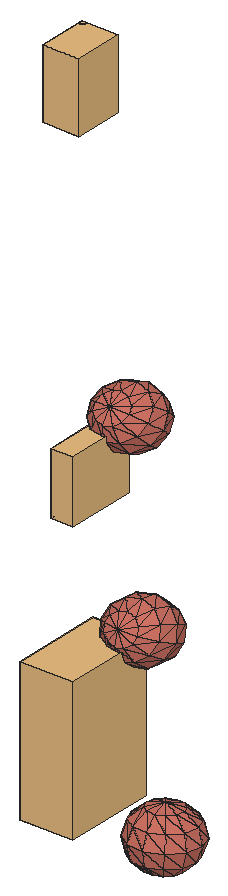
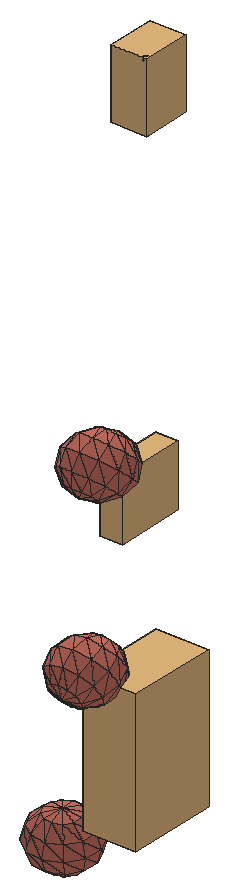
# SketchUp Ruby script. Lengths in inches.
U = 1.inch
M = Sketchup.active_model
def pt(a) = Geom::Point3d.new(a.map { |v| v * U })
def face(e, loops, mat)
  f = e.add_face(loops[0].map { |a| pt(a) })
  loops[1..].each { |l| e.add_face(l.map { |a| pt(a) }).erase! }
  f.material = f.back_material = mat if mat
  f
end
# faces: each face lists its corners as indices into pts; further lists are holes
def faces(e, pts, list, mat = nil) = list.each { |f| face(e, (f[0].is_a?(Array) ? f : [f]).map { |l| l.map { |i| pts[i] } }, mat) }
# xy, xz, yz: faces in a plane at the given z, y or x. An outline is a flat list of corners, or four numbers for a rectangle; further outlines are holes
def ring(l) = l.size == 4 ? [[l[0], l[1]], [l[2], l[1]], [l[2], l[3]], [l[0], l[3]]] : l.each_slice(2).to_a
def flat(e, list, mat, &to3) = list.each { |f| face(e, (f[0].is_a?(Array) ? f : [f]).map { |l| ring(l).map { |u, v| to3.(u, v) } }, mat) }
def xy(e, z, list, mat = nil) = flat(e, list, mat) { |x, y| [x, y, z] }
def xz(e, y, list, mat = nil) = flat(e, list, mat) { |x, z| [x, y, z] }
def yz(e, x, list, mat = nil) = flat(e, list, mat) { |y, z| [x, y, z] }
def lines(e, pts, list) = list.each { |a, b| e.add_line(pt(pts[a]), pt(pts[b])) }
# prism: a flat outline (further loops are holes) pulled along v
def prism(e, loops, v, mat = nil)
  f = face(e, loops, mat); d = Geom::Vector3d.new(v.map { |x| x * U })
  f.pushpull(f.normal.samedirection?(d) ? d.length : -d.length)
end
def box(e, o, s, mat = nil) = prism(e, [[o, [o[0] + s[0], o[1], o[2]], [o[0] + s[0], o[1] + s[1], o[2]], [o[0], o[1] + s[1], o[2]]]], [0, 0, s[2]], mat)
def at(x, y, z, deg = 0) = Geom::Transformation.translation(pt([x, y, z])) * Geom::Transformation.rotation(ORIGIN, Z_AXIS, deg.degrees)
def axes(o, x, y, z) = Geom::Transformation.new([*x, 0, *y, 0, *z, 0, *pt(o).to_a, 1])
def part(name) = M.definitions.add(name)
# library, detail: a bought-in or finely detailed component or shape, given as its bounding box
def library(name, o, s) = part(name).tap { |d| box(d.entities, o, s) }
def detail(e, o, s) = box(e.add_group.entities, o, s)
def put(e, d, t, mat = nil) = e.add_instance(d, t).tap { |i| i.material = mat if mat }
def group(e, t, mat = nil) = e.add_group.tap { |g| g.transformation = t; g.material = mat if mat }.entities
root = M.entities
M.materials.add("green").color = [174, 139, 102]
M.materials.add("vio").color = [206, 114, 100]
c1 = library("3DGeom~25_Defintion",[-351.97,-500,-258.4],[703.94,1000,516.8])
c2 = part("3DGeom~26_Defintion")
p = [[-344.73,487.39,-243.89],[-293.86,494.46,-251.4],[-311.18,491.2,-258.4],[-344.73,487.39,-243.89],[-311.18,491.2,-258.4],[-329.79,488.61,-255.65],
  [-344.73,487.39,-243.89],[-282.49,497.51,-236.53],[-293.86,494.46,-251.4],[-344.73,487.39,-243.89],[-351.97,487.85,-226.26],[-349.59,489.88,-207.5],
  [-344.73,487.39,-243.89],[-349.59,489.88,-207.5],[-338.22,492.93,-192.625],[-344.73,487.39,-243.89],[-280.11,499.54,-217.76],[-282.49,497.51,-236.53],
  [-344.73,487.39,-243.89],[-302.29,498.77,-188.375],[-287.36,500,-200.14],[-344.73,487.39,-243.89],[-287.36,500,-200.14],[-280.11,499.54,-217.76],
  [-344.73,487.39,-243.89],[-338.22,492.93,-192.625],[-320.91,496.1875,-185.625],[-344.73,487.39,-243.89],[-320.91,496.1875,-185.625],[-302.29,498.77,-188.375],
  [300.11,-500,207.2],[314.12,-496.86,194.8],[330.21,-489.05,190.33],[351.97,-468.47,207.5],[300.11,-500,207.2],[330.21,-489.05,190.33],
  [351.97,-468.47,207.5],[330.21,-489.05,190.33],[344.06,-478.66,194.98],[291.79,-490.37,241.23],[300.11,-500,207.2],[313.56,-469.79,258.4],
  [300.11,-500,207.2],[291.79,-490.37,241.23],[291.94,-497.625,224.19],[343.65,-458.84,241.54],[300.11,-500,207.2],[351.97,-468.47,207.5],
  [313.56,-469.79,258.4],[300.11,-500,207.2],[343.65,-458.84,241.54],[343.65,-458.84,241.54],[351.97,-468.47,207.5],[351.82,-461.21,224.54],
  [291.79,-490.37,241.23],[313.56,-469.79,258.4],[299.7,-480.18,253.76],[313.56,-469.79,258.4],[343.65,-458.84,241.54],[329.64,-461.98,253.93]]
faces(c2.entities,p,[[0,1,2],[3,4,5],[6,7,8],[9,10,11],[12,13,14],[15,16,17],[18,19,20],[21,22,23],
  [24,25,26],[27,28,29],[30,31,32],[33,34,35],[36,37,38],[39,40,41],[42,43,44],[45,46,47],
  [48,49,50],[51,52,53],[54,55,56],[57,58,59]],"green")
c3 = library("3DGeom~17_Defintion",[-322.12,-500,-186.09],[644.24,1000,372.18])
c4 = part("3DGeom~18_Defintion")
p = [[292.74,-500,-165.38],[307.55,-495.14,-174.52],[291.14,-497.07,-147.46],[307.55,-495.14,-174.52],[292.74,-500,-165.38],[299.25,-498.4,-172.01],
  [291.14,-497.07,-147.46],[307.55,-495.14,-174.52],[304.35,-489.29,-138.68],[304.35,-489.29,-138.68],[307.55,-495.14,-174.52],[319.15,-484.43,-147.83],
  [307.55,-495.14,-174.52],[315.42,-491.1,-172.22],[320.75,-487.36,-165.74],[320.75,-487.36,-165.74],[319.15,-484.43,-147.83],[320.75,-487.36,-165.74],
  [322.12,-484.92,-156.8125],[292.74,-500,-165.38],[291.14,-497.07,-147.46],[289.78,-499.51,-156.39],[304.35,-489.29,-138.68],[319.15,-484.43,-147.83],
  [312.65,-486.03,-141.19],[291.14,-497.07,-147.46],[304.35,-489.29,-138.68],[296.48,-493.33,-140.98],[-309.07,495.99,151.67],[-322.12,484.07,169.09],
  [-318.39,482.74,177.66],[-309.07,495.99,151.67],[-318.39,482.74,177.66],[-311.33,483.72,183.88],[-309.07,495.99,151.67],[-311.33,483.72,183.88],
  [-302.83,486.75,186.09],[-309.07,495.99,151.67],[-321.51,487.36,160.45],[-322.12,484.07,169.09],[-309.07,495.99,151.67],[-302.83,486.75,186.09],
  [-295.16,491.02,183.67],[-309.07,495.99,151.67],[-316.73,491.72,154.08],[-321.51,487.36,160.45],[-309.07,495.99,151.67],[-295.16,491.02,183.67],
  [-290.38,495.38,177.3],[-309.07,495.99,151.67],[-290.38,495.38,177.3],[-289.78,498.67,168.67],[-309.07,495.99,151.67],[-289.78,498.67,168.67],
  [-293.5,500,160.09],[-309.07,495.99,151.67],[-293.5,500,160.09],[-300.5625,499.02,153.87]]
faces(c4.entities,p,[[0,1,2],[3,4,5],[6,7,8],[9,10,11],[12,13,14],[11,10,15],[16,17,18],[19,20,21],
  [22,23,24],[25,26,27],[28,29,30],[31,32,33],[34,35,36],[37,38,39],[40,41,42],[43,44,45],
  [46,47,48],[49,50,51],[52,53,54],[55,56,57]],"green")
c5 = library("3DGeom~21_Defintion",[-500,-446.39,-160.99],[1000,892.78,321.97])
c6 = part("3DGeom~22_Defintion")
p = [[448.91,-442.9,-142.17],[471.3125,-423.55,-160.99],[450.7,-444.07,-105.16],[450.7,-444.07,-105.16],[471.3125,-423.55,-160.99],[474.89,-425.89,-86.96],
  [471.3125,-423.55,-160.99],[448.91,-442.9,-142.17],[458.1,-434.54,-155.85],[474.89,-425.89,-86.96],[471.3125,-423.55,-160.99],[497.29,-406.54,-105.77],
  [471.3125,-423.55,-160.99],[485,-412.87,-156.2],[495.5,-405.37,-142.78],[471.3125,-423.55,-160.99],[495.5,-405.37,-142.78],[495.5,-405.37,-142.78],
  [500,-403.05,-124.32],[448.91,-442.9,-142.17],[450.7,-444.07,-105.16],[446.2,-446.39,-123.62],[474.89,-425.89,-86.96],[488.1,-414.9,-92.09],
  [450.7,-444.07,-105.16],[474.89,-425.89,-86.96],[461.21,-436.57,-91.74],[-483.76,433.75,98.79],[-496.54,399.82,130.23],[-485.88,396.59,145.74],
  [-483.76,433.75,98.79],[-485.88,396.59,145.74],[-470.87,400.03,156.99],[-483.76,433.75,98.79],[-500,408.86,114.64],[-496.54,399.82,130.23],
  [-483.76,433.75,98.79],[-470.87,400.03,156.99],[-455.53,409.22,160.98],[-483.76,433.75,98.79],[-495.32,421.28,103.125],[-483.76,433.75,98.79],
  [-455.53,409.22,160.98],[-443.97,421.7,156.64],[-483.76,433.75,98.79],[-443.97,421.7,156.64],[-439.29,434.12,145.13],[-483.76,433.75,98.79],
  [-442.75,443.16,129.53],[-453.41,446.39,114.03],[-483.76,433.75,98.79],[-453.41,446.39,114.03],[-468.42,442.95,102.78],[-483.76,433.75,98.79],
  [-439.29,434.12,145.13],[-442.75,443.16,129.53]]
faces(c6.entities,p,[[0,1,2],[3,4,5],[6,7,8],[9,10,11],[12,13,14],[11,15,16],[11,17,18],[19,20,21],
  [22,11,23],[24,25,26],[27,28,29],[30,31,32],[33,34,35],[36,37,38],[39,40,34],[41,42,43],
  [44,45,46],[47,48,49],[50,51,52],[53,54,55]],"green")
c7 = part("3DGeom~225_Defintion")
p = [[77.58,-12.43,-500],[-128.33,-244.69,-395.82],[-181.28,-36.33,-470.68],[95.84,-224,-421.21],[315.65,14.8,-395.34],[38.53,202.47,-444.81],
  [244.7,226.05,-354.18],[-310.44,-256.96,-261.21],[-391.56,-50.49,-315.24],[-310.44,-256.96,-261.21],[-185.65,181.77,-419.42],[-391.56,-50.49,-315.24],
  [-10.85,363.12,-270.44],[108.1875,376.73,-218.11],[-10.85,363.12,-270.44],[108.1875,376.73,-218.11],[-41,-387.49,-214.9],[88.43,-375.54,-229.56],
  [-41,-387.49,-214.9],[302.01,-200.41,-330.58],[-391.56,-50.49,-315.24],[-367.76,169.5,-284.8125],[-140.27,351.16,-255.78],[-367.76,169.5,-284.8125],
  [-10.85,363.12,-270.44],[-140.27,351.16,-255.78],[-128.33,-244.69,-395.82],[-146.14,-394.58,-137.18],[-310.44,-256.96,-261.21],[-128.33,-244.69,-395.82],
  [-41,-387.49,-214.9],[469.13,38.07,-184.76],[302.01,-200.41,-330.58],[315.65,14.8,-395.34],[377.625,246.2,-171.81],[315.65,14.8,-395.34],
  [244.7,226.05,-354.18],[377.625,246.2,-171.81],[315.65,14.8,-395.34],[184.93,388.36,-112.82],[244.7,226.05,-354.18],[108.1875,376.73,-218.11],
  [377.625,246.2,-171.81],[244.7,226.05,-354.18],[207.46,-361.93,-177.23],[434.94,-180.27,-148.2],[207.46,-361.93,-177.23],[302.01,-200.41,-330.58],
  [302.01,-200.41,-330.58],[-391.56,-50.49,-315.24],[-401.6875,-257.51,-53.44],[-496.92,-51.13,-75.34],[-310.44,-256.96,-261.21],[-367.76,169.5,-284.8125],
  [-459,168.95,-77.05],[-245.41,344.08,-178.0625],[-140.27,351.16,-255.78],[-367.76,169.5,-284.8125],[-245.41,344.08,-178.0625],[-10.85,363.12,-270.44],
  [-140.27,351.16,-255.78],[-57.32,426.47,-23.6],[-310.44,-256.96,-261.21],[-198.82,-394.9,-17.23],[-401.6875,-257.51,-53.44],[-310.44,-256.96,-261.21],
  [-245.41,344.08,-178.0625],[88.43,-375.54,-229.56],[57.32,-426.47,23.6],[88.43,-375.54,-229.56],[207.46,-361.93,-177.23],[496.92,51.13,75.34],
  [401.6875,257.51,53.44],[377.625,246.2,-171.81],[401.6875,257.51,53.44],[-245.41,344.08,-178.0625],[-298.1,343.77,-58.11],[-298.1,343.77,-58.11],
  [207.46,-361.93,-177.23],[284.2,-350.3,-71.9375],[284.2,-350.3,-71.9375],[207.46,-361.93,-177.23],[198.82,394.9,17.23],[401.6875,257.51,53.44],
  [459,-168.95,77.05],[-469.13,-38.07,184.76],[-434.94,180.27,148.2],[-298.1,343.77,-58.11],[-377.625,-246.2,171.81],[284.2,-350.3,-71.9375],
  [298.1,-343.77,58.11],[298.1,-343.77,58.11],[-298.1,343.77,-58.11],[-284.2,350.3,71.9375],[-284.2,350.3,71.9375],[-401.6875,-257.51,-53.44],
  [-184.93,-388.36,112.82],[-401.6875,-257.51,-53.44],[-377.625,-246.2,171.81],[-207.46,361.93,177.23],[-88.43,375.54,229.56],[41,387.49,214.9],
  [146.14,394.58,137.18],[-108.1875,-376.73,218.11],[10.85,-363.12,270.44],[-108.1875,-376.73,218.11],[140.27,-351.16,255.78],[10.85,-363.12,270.44],
  [298.1,-343.77,58.11],[245.41,-344.08,178.0625],[245.41,-344.08,178.0625],[140.27,-351.16,255.78],[310.44,256.96,261.21],[401.6875,257.51,53.44],
  [310.44,256.96,261.21],[367.76,-169.5,284.8125],[245.41,-344.08,178.0625],[-284.2,350.3,71.9375],[-302.01,200.41,330.58],[-284.2,350.3,71.9375],
  [-302.01,200.41,330.58],[-207.46,361.93,177.23],[391.56,50.49,315.24],[310.44,256.96,261.21],[-377.625,-246.2,171.81],[-108.1875,-376.73,218.11],
  [-315.65,-14.8,395.34],[-315.65,-14.8,395.34],[-302.01,200.41,330.58],[-377.625,-246.2,171.81],[-108.1875,-376.73,218.11],[-244.7,-226.05,354.18],
  [-244.7,-226.05,354.18],[-207.46,361.93,177.23],[-302.01,200.41,330.58],[-95.84,224,421.21],[-207.46,361.93,177.23],[-88.43,375.54,229.56],
  [185.65,-181.77,419.42],[140.27,-351.16,255.78],[245.41,-344.08,178.0625],[245.41,-344.08,178.0625],[367.76,-169.5,284.8125],[-244.7,-226.05,354.18],
  [-315.65,-14.8,395.34],[-88.43,375.54,229.56],[128.33,244.69,395.82],[41,387.49,214.9],[128.33,244.69,395.82],[-244.7,-226.05,354.18],
  [-108.1875,-376.73,218.11],[10.85,-363.12,270.44],[-88.43,375.54,229.56],[128.33,244.69,395.82],[-38.53,-202.47,444.81],[128.33,244.69,395.82],
  [391.56,50.49,315.24],[310.44,256.96,261.21],[181.28,36.33,470.68],[367.76,-169.5,284.8125],[367.76,-169.5,284.8125],[391.56,50.49,315.24],
  [128.33,244.69,395.82],[391.56,50.49,315.24],[-315.65,-14.8,395.34],[-77.58,12.43,500],[128.33,244.69,395.82]]
faces(c7.entities,p,[[0,1,2],[0,3,1],[4,3,0],[5,0,2],[6,0,5],[6,4,0],[2,7,8],[2,1,9],
  [10,2,11],[5,2,10],[12,5,10],[13,5,14],[15,6,5],[3,16,1],[3,17,18],[19,17,3],
  [4,19,3],[10,20,21],[22,10,23],[24,10,25],[26,27,28],[29,30,27],[31,32,33],[34,35,36],
  [37,31,38],[39,40,41],[39,42,43],[19,44,17],[45,46,47],[31,45,48],[49,50,51],[49,52,50],
  [53,49,51],[53,51,54],[55,53,54],[56,57,58],[59,60,61],[41,59,61],[62,63,64],[65,27,63],
  [60,66,61],[30,67,68],[69,70,68],[39,41,61],[27,30,68],[71,45,31],[72,31,73],[74,71,31],
  [75,54,76],[66,77,61],[78,79,68],[45,80,81],[82,42,39],[82,83,42],[84,80,45],[71,84,45],
  [63,27,68],[82,39,61],[54,51,85],[54,85,86],[87,54,86],[51,50,88],[51,88,85],[89,90,68],
  [84,91,80],[92,86,93],[77,94,61],[95,63,96],[97,96,98],[94,99,61],[99,100,61],[100,101,61],
  [101,102,61],[102,82,61],[96,63,68],[102,83,82],[103,96,68],[104,105,68],[106,107,68],[108,109,68],
  [110,111,68],[112,71,113],[102,114,83],[115,116,91],[115,91,84],[117,86,118],[119,120,121],[122,84,71],
  [123,122,71],[122,115,84],[124,96,125],[101,114,102],[86,85,126],[86,127,128],[129,130,131],[85,88,132],
  [133,134,135],[136,135,137],[138,139,140],[138,141,142],[85,143,144],[145,146,147],[101,148,114],[149,150,151],
  [152,135,153],[154,151,139],[154,139,138],[155,156,157],[149,151,154],[158,138,159],[158,160,161],[162,158,163],
  [134,164,165],[134,165,135],[164,149,154],[164,154,165],[135,158,166],[165,154,138],[165,138,158],[135,165,158]],"vio")
c8 = part("3DGeom~195_Defintion")
p = [[166.45,-153.95,-435.25],[-186.98,-146.09,-430.65],[-6.51,0,-500],[325.5,12.77,-379.3],[-335.26,-12.77,-370.7],[-177.72,153.95,-430.77],
  [175.71,146.09,-435.37],[397.32,176.07,-221.71],[27.43,279.42,-375.42],[310.84,253.04,-254.09],[27.43,279.42,-375.42],[397.32,176.07,-221.71],
  [310.84,253.04,-254.09],[-37.19,-279.42,-374.58],[294.8125,-266.65,-253.88],[436.66,-84.83,-222.23],[436.66,-84.83,-222.23],[-442.29,84.83,-210.79],
  [-442.29,84.83,-210.79],[-301.32,266.65,-246.12],[27.43,279.42,-375.42],[-301.32,266.65,-246.12],[-317.35,-253.04,-245.91],[-402.96,-176.07,-211.3],
  [-402.96,-176.07,-211.3],[461.5,119.72,-131.03],[436.66,-84.83,-222.23],[325.5,12.77,-379.3],[325.5,12.77,-379.3],[397.32,176.07,-221.71],
  [310.84,253.04,-254.09],[27.43,279.42,-375.42],[225.23,330.02,-219.47],[27.43,279.42,-375.42],[-301.32,266.65,-246.12],[-79.61,377.03,-215.51],
  [225.23,330.02,-219.47],[27.43,279.42,-375.42],[-79.61,377.03,-215.51],[73.97,-377.02,-217.51],[-230.87,-330.02,-213.54],[-37.19,-279.42,-374.58],
  [73.97,-377.02,-217.51],[-230.87,-330.02,-213.54],[-335.26,-12.77,-370.7],[-402.96,-176.07,-211.3],[-464.76,-119.72,-118.97],[-335.26,-12.77,-370.7],
  [-442.29,84.83,-210.79],[310.84,253.04,-254.09],[362.6875,292.19,-4.72],[225.23,330.02,-219.47],[344.18,-307.91,-4.48],[73.97,-377.02,-217.51],
  [294.8125,-266.65,-253.88],[479.41,-120.56,-6.24],[344.18,-307.91,-4.48],[294.8125,-266.65,-253.88],[294.8125,-266.65,-253.88],[-301.32,266.65,-246.12],
  [-479.41,120.56,6.24],[-301.32,266.65,-246.12],[-344.18,307.91,4.48],[-301.32,266.65,-246.12],[-344.18,307.91,4.48],[-317.35,-253.04,-245.91],
  [-230.87,-330.02,-213.54],[-362.6875,-292.19,4.72],[-317.35,-253.04,-245.91],[-362.6875,-292.19,4.72],[486.1875,99.09,-6.33],[163.4375,386.37,-127.15],
  [362.6875,292.19,-4.72],[116.72,-412.75,-1.52],[-166.69,-386.37,-122.85],[73.97,-377.02,-217.51],[344.18,-307.91,-4.48],[73.97,-377.02,-217.51],
  [73.97,-377.02,-217.51],[-230.87,-330.02,-213.54],[-116.72,412.75,1.52],[-230.87,-330.02,-213.54],[-362.6875,-292.19,4.72],[-362.6875,-292.19,4.72],
  [-486.1875,-99.09,6.33],[142.01,407,-1.85],[362.6875,292.19,-4.72],[-142.01,-407,1.85],[-362.6875,-292.19,4.72],[464.76,119.72,118.97],
  [442.29,-84.83,210.79],[402.96,176.07,211.3],[317.35,253.04,245.91],[230.87,330.02,213.54],[166.69,386.37,122.85],[362.6875,292.19,-4.72],
  [230.87,330.02,213.54],[362.6875,292.19,-4.72],[301.32,-266.65,246.12],[344.18,-307.91,-4.48],[301.32,-266.65,246.12],[-73.97,377.02,217.51],
  [79.61,-377.03,215.51],[301.32,-266.65,246.12],[-294.8125,266.65,253.88],[-294.8125,266.65,253.88],[-163.4375,-386.37,127.15],[-344.18,307.91,4.48],
  [-436.66,84.83,222.23],[-344.18,307.91,4.48],[-436.66,84.83,222.23],[-294.8125,266.65,253.88],[-225.24,-330.02,219.47],[-225.24,-330.02,219.47],
  [-310.84,-253.04,254.09],[-362.6875,-292.19,4.72],[-461.5,-119.72,131.03],[-362.6875,-292.19,4.72],[-397.32,-176.07,221.71],[-362.6875,-292.19,4.72],
  [-310.84,-253.04,254.09],[-397.32,-176.07,221.71],[-362.6875,-292.19,4.72],[-436.66,84.83,222.23],[37.19,279.42,374.58],[37.19,279.42,374.58],
  [230.87,330.02,213.54],[-27.43,-279.42,375.42],[-27.43,-279.42,375.42],[-436.66,84.83,222.23],[-397.32,-176.07,221.71],[335.26,12.77,370.7],
  [301.32,-266.65,246.12],[442.29,-84.83,210.79],[335.26,12.77,370.7],[317.35,253.04,245.91],[335.26,12.77,370.7],[402.96,176.07,211.3],
  [230.87,330.02,213.54],[37.19,279.42,374.58],[186.98,146.09,430.65],[230.87,330.02,213.54],[317.35,253.04,245.91],[177.72,-153.95,430.77],
  [-27.43,-279.42,375.42],[79.61,-377.03,215.51],[79.61,-377.03,215.51],[301.32,-266.65,246.12],[-73.97,377.02,217.51],[-294.8125,266.65,253.88],
  [-166.45,153.95,435.25],[-73.97,377.02,217.51],[-175.71,-146.09,435.37],[-310.84,-253.04,254.09],[-225.24,-330.02,219.47],[-225.24,-330.02,219.47],
  [-325.5,-12.77,379.3],[-397.32,-176.07,221.71],[-436.66,84.83,222.23],[-397.32,-176.07,221.71],[-325.5,-12.77,379.3],[-436.66,84.83,222.23],
  [317.35,253.04,245.91],[335.26,12.77,370.7],[335.26,12.77,370.7],[301.32,-266.65,246.12],[335.26,12.77,370.7],[6.51,0,500]]
faces(c8.entities,p,[[0,1,2],[3,0,2],[2,1,4],[2,4,5],[6,2,5],[3,2,6],[7,3,6],[6,5,8],
  [9,6,10],[11,6,12],[0,13,1],[14,13,0],[15,14,0],[16,0,3],[5,4,17],[5,18,19],
  [20,5,21],[13,22,1],[1,22,23],[1,24,4],[25,26,27],[25,28,29],[30,31,32],[33,34,35],
  [36,37,38],[39,40,41],[14,42,13],[13,43,22],[44,45,46],[47,46,48],[29,49,50],[49,51,50],
  [52,53,54],[55,56,57],[55,58,26],[59,48,60],[61,60,62],[38,63,64],[65,66,67],[45,68,69],
  [70,55,26],[70,26,25],[25,29,50],[36,71,72],[36,38,71],[73,74,75],[76,73,77],[78,74,79],
  [38,64,80],[71,38,80],[81,74,82],[46,45,83],[48,46,84],[48,84,60],[70,25,50],[71,85,86],
  [71,80,85],[73,87,74],[74,87,82],[84,46,88],[89,55,70],[89,70,50],[90,56,55],[89,90,55],
  [91,89,50],[92,91,50],[93,92,50],[85,94,95],[94,96,97],[98,73,99],[90,100,56],[85,80,101],
  [85,101,94],[102,87,73],[103,102,73],[80,64,104],[80,105,101],[87,106,82],[102,106,87],[107,60,108],
  [109,110,111],[106,112,82],[113,114,115],[116,84,117],[118,116,119],[120,121,122],[60,84,116],[60,116,123],
  [91,90,89],[94,101,124],[94,125,126],[127,112,106],[128,106,102],[129,116,130],[131,132,133],[91,134,90],
  [135,136,137],[138,139,140],[141,140,142],[143,144,145],[143,146,147],[148,149,150],[151,150,139],[152,153,154],
  [152,155,144],[156,157,153],[158,159,160],[149,161,156],[162,140,163],[164,143,165],[149,156,150],[156,153,152],
  [140,143,166],[139,150,167],[139,167,140],[167,152,144],[167,144,143],[150,156,152],[140,167,143],[150,152,167]],"vio")
c9 = part("3DGeom~193_Defintion")
p = [[111.73,-187.4,-434.54],[-226.37,-99.64,-430.14],[-6.51,0,-500],[317.5,-62.65,-379.2],[-327.26,62.65,-370.81],[215.1,99.64,-435.89],
  [-123,187.4,-431.49],[438.19,78.88,-222.25],[438.19,78.88,-222.25],[379.08,172.58,-254.98],[114.21,261.93,-376.55],[379.08,172.58,-254.98],
  [114.21,261.93,-376.55],[200.03,-324.58,-252.65],[-123.97,-261.93,-373.45],[393.97,-181.45,-221.67],[393.97,-181.45,-221.67],[-399.61,181.45,-211.34],
  [-399.61,181.45,-211.34],[-206.54,324.58,-247.35],[114.21,261.93,-376.55],[-206.54,324.58,-247.35],[-385.58,-172.58,-245.02],[-226.37,-99.64,-430.14],
  [-385.58,-172.58,-245.02],[-443.83,-78.88,-210.77],[-226.37,-99.64,-430.14],[-327.26,62.65,-370.81],[482.35,10.29,-131.3],[393.97,-181.45,-221.67],
  [317.5,-62.65,-379.2],[317.5,-62.65,-379.2],[438.19,78.88,-222.25],[379.08,172.58,-254.98],[114.21,261.93,-376.55],[320.83,266.28,-220.72],
  [114.21,261.93,-376.55],[-206.54,324.58,-247.35],[41.87,380.73,-217.09],[320.83,266.28,-220.72],[114.21,261.93,-376.55],[41.87,380.73,-217.09],
  [-47.5,-380.73,-215.93],[-326.46,-266.28,-212.3],[-123.97,-261.93,-373.45],[-47.5,-380.73,-215.93],[-326.46,-266.28,-212.3],[-385.58,-172.58,-245.02],
  [-327.26,62.65,-370.81],[-485.6,-10.29,-118.7],[-327.26,62.65,-370.81],[-399.61,181.45,-211.34],[379.08,172.58,-254.98],[441.47,199.28,-5.74],
  [320.83,266.28,-220.72],[234.74,-374.79,-3.05],[-47.5,-380.73,-215.93],[200.03,-324.58,-252.65],[424.02,-224.9375,-5.52],[234.74,-374.79,-3.05],
  [200.03,-324.58,-252.65],[200.03,-324.58,-252.65],[-206.54,324.58,-247.35],[-424.02,224.9375,5.52],[-206.54,324.58,-247.35],[-234.74,374.79,3.05],
  [-206.54,324.58,-247.35],[-234.74,374.79,3.05],[-326.46,-266.28,-212.3],[-441.47,-199.28,5.74],[499.7,-14.8125,-6.5],[279.06,334.87,-128.65],
  [320.83,266.28,-220.72],[279.06,334.87,-128.65],[279.06,334.87,-128.65],[17.45,424.22,-0.23],[-17.45,-424.22,0.23],[-282.3125,-334.87,-121.35],
  [-47.5,-380.73,-215.93],[234.74,-374.79,-3.05],[-47.5,-380.73,-215.93],[-47.5,-380.73,-215.93],[-326.46,-266.28,-212.3],[-326.46,-266.28,-212.3],
  [-282.3125,-334.87,-121.35],[-499.7,14.8125,6.5],[264.96,359.98,-3.45],[279.06,334.87,-128.65],[264.96,359.98,-3.45],[-264.96,-359.98,3.45],
  [-282.3125,-334.87,-121.35],[-264.96,-359.98,3.45],[485.6,10.29,118.7],[443.83,78.88,210.77],[385.58,172.58,245.02],[326.46,266.28,212.3],
  [282.3125,334.87,121.35],[399.61,-181.45,211.34],[264.96,359.98,-3.45],[47.5,380.73,215.93],[282.3125,334.87,121.35],[264.96,359.98,-3.45],
  [206.54,-324.58,247.36],[234.74,-374.79,-3.05],[206.54,-324.58,247.36],[-200.03,324.58,252.65],[-200.03,324.58,252.65],[-41.87,-380.73,217.09],
  [206.54,-324.58,247.36],[-234.74,374.79,3.05],[-393.97,181.45,221.67],[-234.74,374.79,3.05],[-393.97,181.45,221.67],[-200.03,324.58,252.65],
  [-279.06,-334.87,128.65],[-264.96,-359.98,3.45],[-279.06,-334.87,128.65],[-482.35,-10.29,131.3],[-393.97,181.45,221.67],[-279.06,-334.87,128.65],
  [-320.83,-266.28,220.72],[-320.83,-266.28,220.72],[-379.08,-172.58,254.98],[-438.19,-78.88,222.25],[-379.08,-172.58,254.98],[-438.19,-78.88,222.25],
  [282.3125,334.87,121.35],[123.97,261.93,373.45],[282.3125,334.87,121.35],[123.97,261.93,373.45],[326.46,266.28,212.3],[-114.21,-261.93,376.55],
  [-114.21,-261.93,376.55],[-320.83,-266.28,220.72],[-393.97,181.45,221.67],[-438.19,-78.88,222.25],[327.26,-62.65,370.81],[327.26,-62.65,370.81],
  [206.54,-324.58,247.36],[399.61,-181.45,211.34],[326.46,266.28,212.3],[123.97,261.93,373.45],[226.37,99.64,430.14],[326.46,266.28,212.3],
  [226.37,99.64,430.14],[385.58,172.58,245.02],[47.5,380.73,215.93],[-200.03,324.58,252.65],[-111.73,187.4,434.54],[47.5,380.73,215.93],
  [123,-187.4,431.49],[-114.21,-261.93,376.55],[-41.87,-380.73,217.09],[-41.87,-380.73,217.09],[206.54,-324.58,247.36],[-215.1,-99.64,435.89],
  [-379.08,-172.58,254.98],[-320.83,-266.28,220.72],[-320.83,-266.28,220.72],[-393.97,181.45,221.67],[-438.19,-78.88,222.25],[-317.5,62.65,379.2],
  [-393.97,181.45,221.67],[-317.5,62.65,379.2],[-438.19,-78.88,222.25],[226.37,99.64,430.14],[327.26,-62.65,370.81],[206.54,-324.58,247.36],
  [226.37,99.64,430.14],[327.26,-62.65,370.81],[6.51,0,500],[226.37,99.64,430.14],[226.37,99.64,430.14]]
faces(c9.entities,p,[[0,1,2],[3,0,2],[2,1,4],[3,2,5],[2,4,6],[5,2,6],[7,3,5],[8,5,9],
  [5,6,10],[11,5,12],[13,14,0],[15,13,0],[0,14,1],[16,0,3],[6,4,17],[6,18,19],
  [20,6,21],[14,22,1],[23,24,25],[26,25,27],[28,29,30],[28,31,32],[33,34,35],[36,37,38],
  [39,40,41],[42,43,44],[13,45,14],[14,46,47],[48,25,49],[50,49,51],[32,52,53],[52,54,53],
  [55,56,57],[58,59,60],[58,61,29],[62,51,63],[64,63,65],[41,66,67],[24,68,69],[25,24,69],
  [28,32,53],[70,58,29],[70,29,28],[54,71,53],[72,41,73],[74,41,75],[41,67,75],[76,77,78],
  [79,76,80],[81,77,82],[83,84,69],[51,49,85],[51,85,63],[49,25,69],[70,28,53],[71,86,53],
  [87,75,88],[76,89,77],[90,91,69],[85,49,69],[92,58,70],[92,70,53],[93,92,53],[94,93,53],
  [95,94,53],[86,96,53],[96,95,53],[97,59,58],[92,97,58],[98,99,100],[101,75,99],[102,76,103],
  [97,104,59],[75,67,105],[75,106,99],[107,89,76],[108,107,76],[109,63,110],[111,112,113],[107,114,89],
  [115,116,69],[63,85,117],[63,117,118],[119,120,69],[121,122,69],[117,85,69],[123,117,69],[124,125,69],
  [93,97,92],[126,99,127],[128,129,130],[131,114,107],[132,133,114],[134,117,135],[93,136,97],[94,136,93],
  [137,138,139],[140,141,142],[143,144,145],[146,147,148],[149,148,141],[150,151,152],[150,153,154],[155,156,157],
  [155,158,151],[159,160,161],[147,162,163],[163,164,156],[94,165,136],[166,150,167],[147,163,148],[163,156,155],
  [168,150,169],[141,148,170],[141,170,171],[170,155,151],[170,151,150],[148,163,155],[172,170,150],[148,155,170]],"vio")
g1 = group(root,at(15.3125,134.49,26.21))
put(g1,c1,axes([3.34,0.21,15.8],[0,0.0004,0],[0,0,-0.0004],[-0.0004,0,0]),"green")
put(g1,c2,axes([3.34,0.21,15.8],[0,0.0004,0],[0,0,-0.0004],[-0.0004,0,0]),"green")
g2 = group(root,at(15.3125,134.49,26.21))
put(g2,c3,axes([3.3125,0.26,12.43],[0,0.00081,0],[0,0,-0.00081],[-0.00081,0,0]),"green")
put(g2,c4,axes([3.3125,0.26,12.43],[0,0.00081,0],[0,0,-0.00081],[-0.00081,0,0]),"green")
g3 = group(root,at(15.3125,134.49,26.21))
put(g3,c5,axes([3.32,0.3,13.74],[0,0.0004,0],[0,0,-0.0004],[-0.0004,0,0]),"green")
put(g3,c6,axes([3.32,0.3,13.74],[0,0.0004,0],[0,0,-0.0004],[-0.0004,0,0]),"green")
g4 = group(root,at(15.3125,134.49,26.21))
put(g4,c7,axes([3.63,0.45,11.9],[0,0.00039,0],[0,0,-0.00039],[-0.00039,0,0]),"vio")
g5 = group(root,at(15.3125,134.49,26.21))
put(g5,c8,axes([3.375,0.52,13.9375],[0,0.00039,0],[0,0,-0.00039],[-0.00039,0,0]),"vio")
g6 = group(root,at(15.3125,134.49,26.21))
put(g6,c9,axes([3.44,0.53,12.86],[0,0.00039,0],[0,0,-0.00039],[-0.00039,0,0]),"vio")
